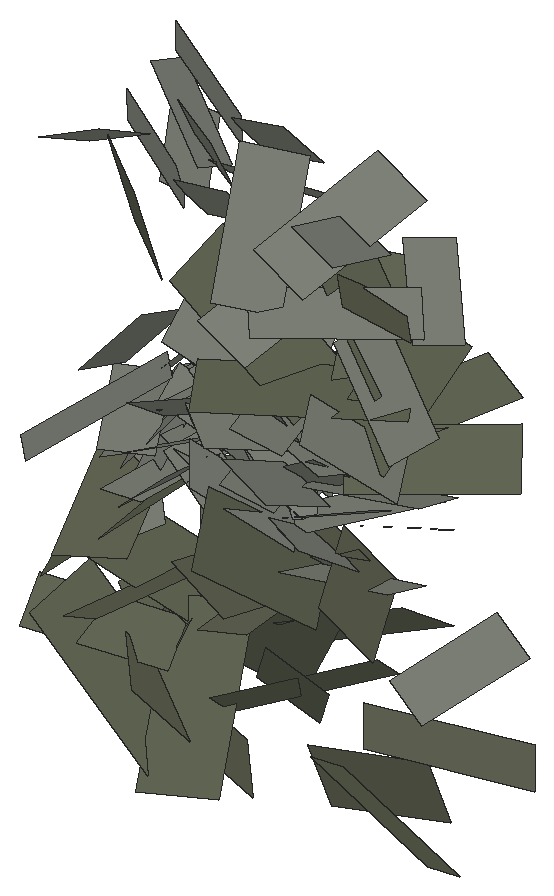
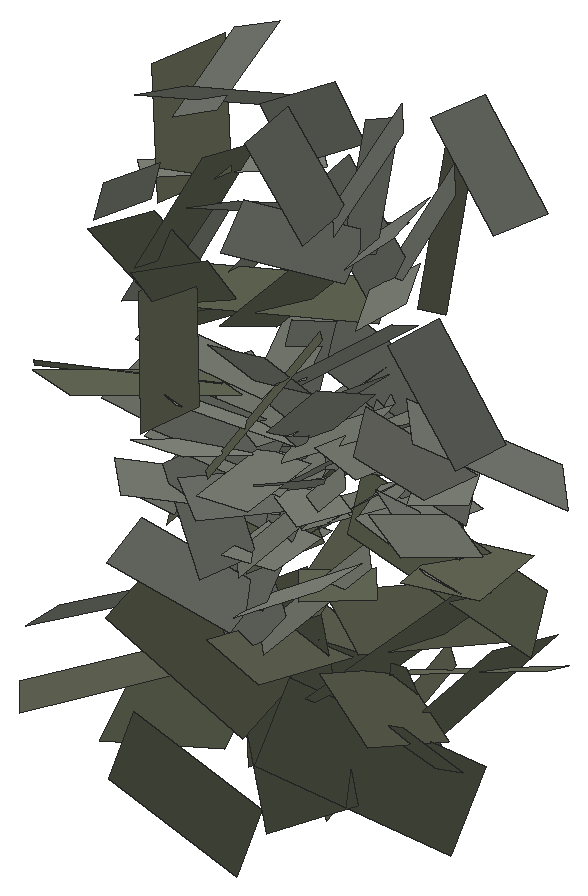
# SketchUp Ruby script. Lengths in inches.
U = 1.inch
M = Sketchup.active_model
def pt(a) = Geom::Point3d.new(a.map { |v| v * U })
def face(e, loops, mat)
  f = e.add_face(loops[0].map { |a| pt(a) })
  loops[1..].each { |l| e.add_face(l.map { |a| pt(a) }).erase! }
  f.material = f.back_material = mat if mat
  f
end
# faces: each face lists its corners as indices into pts; further lists are holes
def faces(e, pts, list, mat = nil) = list.each { |f| face(e, (f[0].is_a?(Array) ? f : [f]).map { |l| l.map { |i| pts[i] } }, mat) }
# xy, xz, yz: faces in a plane at the given z, y or x. An outline is a flat list of corners, or four numbers for a rectangle; further outlines are holes
def ring(l) = l.size == 4 ? [[l[0], l[1]], [l[2], l[1]], [l[2], l[3]], [l[0], l[3]]] : l.each_slice(2).to_a
def flat(e, list, mat, &to3) = list.each { |f| face(e, (f[0].is_a?(Array) ? f : [f]).map { |l| ring(l).map { |u, v| to3.(u, v) } }, mat) }
def xy(e, z, list, mat = nil) = flat(e, list, mat) { |x, y| [x, y, z] }
def xz(e, y, list, mat = nil) = flat(e, list, mat) { |x, z| [x, y, z] }
def yz(e, x, list, mat = nil) = flat(e, list, mat) { |y, z| [x, y, z] }
def lines(e, pts, list) = list.each { |a, b| e.add_line(pt(pts[a]), pt(pts[b])) }
# prism: a flat outline (further loops are holes) pulled along v
def prism(e, loops, v, mat = nil)
  f = face(e, loops, mat); d = Geom::Vector3d.new(v.map { |x| x * U })
  f.pushpull(f.normal.samedirection?(d) ? d.length : -d.length)
end
def box(e, o, s, mat = nil) = prism(e, [[o, [o[0] + s[0], o[1], o[2]], [o[0] + s[0], o[1] + s[1], o[2]], [o[0], o[1] + s[1], o[2]]]], [0, 0, s[2]], mat)
def at(x, y, z, deg = 0) = Geom::Transformation.translation(pt([x, y, z])) * Geom::Transformation.rotation(ORIGIN, Z_AXIS, deg.degrees)
def axes(o, x, y, z) = Geom::Transformation.new([*x, 0, *y, 0, *z, 0, *pt(o).to_a, 1])
def part(name) = M.definitions.add(name)
# library, detail: a bought-in or finely detailed component or shape, given as its bounding box
def library(name, o, s) = part(name).tap { |d| box(d.entities, o, s) }
def detail(e, o, s) = box(e.add_group.entities, o, s)
def put(e, d, t, mat = nil) = e.add_instance(d, t).tap { |i| i.material = mat if mat }
def group(e, t, mat = nil) = e.add_group.tap { |g| g.transformation = t; g.material = mat if mat }.entities
root = M.entities
M.materials.add("viburnumblaasdfas0df1w06d").color = [98, 102, 84]
M.materials.add("viburnumbladsadfasdfad0w122").color = [125, 129, 119]
c1 = part("Component\#315")
p = [[0.25,0,0],[2.05,0.01,0.35],[1.81,4.2,1.66],[0,4.19,1.3125]]
faces(c1.entities,p,[[0,1,2,3]],"viburnumbladsadfasdfad0w122")
c2 = part("viburnumblad2")
put(c2.entities,c1,axes([-19.23,-4.49,-32.18],[83.35428,0,0],[0,79.38502,0],[0,0,83.35428]))
c3 = part("Component\#314")
p = [[0.14,0,0],[2.58,0.05,0.25],[2.44,5.11,2.64],[0,5.05,2.39]]
faces(c3.entities,p,[[0,1,2,3]],"viburnumblaasdfas0df1w06d")
c4 = part("viburnumblad1\#2")
put(c4.entities,c3,axes([-37.25,6.23,19.31],[75.98784,0,0],[0,65.50676,0],[0,0,75.98784]))
put(root,c2,axes([1228.44,286.27,16.52],[0.01089,-0.00213,0.00325],[0.002,0.01232,0.0014],[-0.00372,-0.00076,0.01198]))
put(root,c2,axes([1227.97,286.51,28.15],[-0.00597,-0.01037,0.00113],[0.01154,-0.00613,0.0032],[-0.00222,0.00293,0.01099]))
put(root,c2,axes([1226.95,284.02,17.86],[0.01077,-0.01075,-0.00083],[0.01118,0.01095,0.00335],[-0.00168,-0.00283,0.01488]))
put(root,c2,axes([1230.21,287.73,26.82],[0.00649,0.00565,-0.00743],[-0.0085,0.00924,-0.00029],[0.00584,0.00584,0.00823]))
put(root,c4,axes([1229.8,282.66,14.06],[0.01294,0.00473,-0.00003],[-0.00539,0.01473,-0.00308],[-0.00088,0.0025,0.01352]))
put(root,c2,axes([1230.28,285.14,14.39],[0.0081,0.00545,0.00286],[-0.00642,0.00891,0.00123],[-0.00184,-0.00279,0.01054]))
put(root,c4,axes([1232.59,285.2,10],[-0.00341,0.01096,0.00392],[-0.01337,-0.00302,-0.00319],[-0.00164,-0.0045,0.01114]))
put(root,c2,axes([1230.37,283.98,18.52],[0.01038,0.0062,-0.0034],[-0.00717,0.01088,-0.00204],[0.00185,0.00346,0.01194]))
put(root,c2,axes([1231.46,287.4,26.4],[-0.00945,0.00892,-0.00145],[-0.0064,-0.00533,0.00736],[0.00487,0.007,0.00802]))
put(root,c2,axes([1231.55,287.99,27.68],[-0.00099,0.0108,-0.00603],[-0.01031,0.00186,0.00471],[0.00538,0.00602,0.00839]))
put(root,c2,axes([1228.79,287.2,19.83],[-0.00259,-0.01229,0.00001],[0.0107,-0.00225,0.00618],[-0.00604,0.00128,0.01094]))
put(root,c2,axes([1228.44,287.14,17.97],[0.0062,-0.01038,0.0034],[0.00931,0.00714,0.00482],[-0.00586,0.00014,0.01111]))
put(root,c4,axes([1232.05,286.2,7.57],[0.00865,0.00658,0.00734],[-0.00992,0.01145,0.00143],[-0.0049,-0.0056,0.0108]))
put(root,c4,axes([1227.57,284.9375,12.29],[0.0081,-0.01447,0.00211],[0.01627,0.00971,0.00411],[-0.00412,0.00005,0.0162]))
put(root,c2,axes([1229.75,285.68,15.67],[0.01032,-0.0026,0.00299],[0.00135,0.01024,0.00424],[-0.00373,-0.00356,0.00978]))
put(root,c4,axes([1230.71,285.7,8.77],[0.01224,-0.00166,0.00834],[0.00122,0.01717,0.00163],[-0.00844,-0.00056,0.01227]))
put(root,c4,axes([1230.86,286.15,23.78],[-0.01166,0.00571,0.00452],[-0.00151,-0.01177,0.01017],[0.0071,0.00732,0.00793]))
put(root,c4,axes([1233.14,284.03,6.07],[0.00022,0.01682,0.00237],[-0.01794,-0.00091,0.00812],[0.00704,-0.00224,0.0153]))
put(root,c4,axes([1228.48,287.45,6.375],[0.00095,-0.01143,0.01095],[0.01752,0.00456,0.00324],[-0.00472,0.01026,0.01113]))
put(root,c4,axes([1233.08,288.2,9.65],[-0.00358,0.0126,0.00711],[-0.01496,-0.00708,0.005],[0.00656,-0.00511,0.01237]))
put(root,c2,axes([1232.67,288.93,28.52],[-0.00905,0.00854,-0.00139],[-0.00711,-0.00593,0.00818],[0.00487,0.007,0.00802]))
put(root,c2,axes([1230.2,284.41,16.75],[0.01283,-0.0027,-0.00001],[0.00224,0.01066,-0.00301],[0.0007,0.00327,0.01211]))
put(root,c2,axes([1229.92,285.9375,17.31],[0.00604,-0.00926,0.00001],[0.00806,0.00526,0.00544],[-0.00456,-0.00296,0.00963]))
put(root,c4,axes([1229.6,283.08,11.54],[0.01155,-0.00606,0.00446],[0.00831,0.01316,-0.00362],[-0.00229,0.00493,0.01266]))
put(root,c2,axes([1230.25,285.44,19.69],[0.01229,-0.00259,-0.00001],[0.00249,0.01185,-0.00335],[0.0007,0.00327,0.01211]))
put(root,c2,axes([1232.37,288.87,26.84],[-0.01181,0.00128,0.00407],[0.00154,-0.01046,0.00743],[0.00382,0.0075,0.00815]))
put(root,c2,axes([1230.95,286.21,16.21],[-0.00178,-0.0105,-0.00298],[0.00981,-0.00286,0.00422],[-0.00478,-0.00196,0.00978]))
put(root,c2,axes([1230.54,285.33,17.9375],[0.007,-0.00987,0.00339],[0.00957,0.00618,-0.0018],[-0.00027,0.0039,0.01194]))
put(root,c2,axes([1234.54,289.21,14.47],[0.00007,0.01222,-0.00309],[-0.01226,0.00091,0.00331],[0.0034,0.00296,0.01177]))
put(root,c2,axes([1231.44,288.74,25.56],[-0.00734,-0.00647,0.00686],[0.01022,-0.00834,0.00267],[0.00284,0.00722,0.00872]))
put(root,c4,axes([1233.8,285.51,13.37],[0.00989,0.00806,-0.00127],[-0.00946,0.01134,-0.00169],[0.00005,0.00193,0.01267]))
put(root,c4,axes([1234.6,286.67,5.19],[-0.01033,0.0106,0.00208],[-0.0106,-0.01173,0.00714],[0.00578,0.00298,0.01347]))
put(root,c2,axes([1234.88,287.15,17.48],[-0.00324,0.01089,0.00211],[-0.01127,-0.00408,0.00376],[0.00428,-0.00101,0.01177]))
put(root,c2,axes([1235.0625,286.23,16.13],[-0.00179,0.01029,-0.00409],[-0.01223,-0.00094,0.00298],[0.00221,0.00457,0.01052]))
put(root,c2,axes([1235.05,287.08,18.96],[-0.00186,0.01072,-0.00426],[-0.01132,-0.00087,0.00276],[0.00221,0.00457,0.01052]))
put(root,c4,axes([1233.03,283.23,5.98],[0.01503,0.00487,0.00033],[-0.00521,0.01551,0.00826],[0.00191,-0.00687,0.0141]))
put(root,c2,axes([1234.36,286.95,19.07],[0.00616,0.01091,0.00086],[-0.01009,0.00525,0.00563],[0.00448,-0.00342,0.01123]))
put(root,c2,axes([1235.2,289.14,12.91],[-0.0083,0.00785,-0.00197],[-0.00857,-0.00783,0.00492],[0.002,0.00498,0.01141]))
put(root,c2,axes([1234.42,286.84,17.47],[0.00682,0.00858,-0.00405],[-0.00975,0.00742,-0.00069],[0.00196,0.0036,0.01094]))
put(root,c2,axes([1231.69,285.99,19.34],[-0.00239,-0.01136,0.0048],[0.01232,-0.002,0.0014],[-0.0005,0.00498,0.01153]))
put(root,c2,axes([1231.43,289.91,26.63],[0.00099,-0.0108,0.00603],[0.0122,-0.00051,-0.00294],[0.0025,0.00634,0.00938]))
put(root,c2,axes([1235.61,285.54,14.84],[-0.00037,0.01298,-0.00224],[-0.01317,0.00059,0.00559],[0.0056,0.0024,0.01296]))
put(root,c2,axes([1235.53,289.9,15.8125],[-0.00876,0.00902,-0.0009],[-0.00857,-0.00783,0.00492],[0.00296,0.00403,0.01157]))
put(root,c2,axes([1235.57,286.57,20.35],[-0.00304,0.01166,0.00355],[-0.01127,-0.00408,0.00376],[0.00464,-0.00228,0.01145]))
put(root,c2,axes([1232.8,290.25,27.68],[-0.00765,-0.00673,0.00714],[0.00947,-0.00772,0.00247],[0.00284,0.00722,0.00872]))
put(root,c4,axes([1232.87,290.7,6.53],[-0.01405,-0.00766,0.00571],[0.01107,-0.01374,0.00878],[0.00057,0.00947,0.0141]))
put(root,c2,axes([1235.74,286.91,17.37],[-0.00945,0.00658,-0.00199],[-0.00667,-0.00798,0.00533],[0.00164,0.00544,0.01021]))
put(root,c4,axes([1233.21,285.82,11.08],[0.01241,-0.00186,0.00262],[0.00291,0.01409,-0.00376],[-0.00201,0.00365,0.01212]))
put(root,c2,axes([1235.13,286.12,16.61],[0.00988,0.00976,-0.00351],[-0.00912,0.01058,0.00376],[0.00511,-0.00035,0.01338]))
put(root,c2,axes([1233.9375,287.17,15.875],[0.01201,0.00148,-0.00152],[-0.00157,0.01006,-0.00263],[0.00104,0.00309,0.01122]))
put(root,c2,axes([1234.02,288.09,18.62],[0.01151,0.00142,-0.00146],[-0.00175,0.01118,-0.00292],[0.00104,0.00309,0.01122]))
put(root,c4,axes([1234.72,288.91,12.13],[-0.01223,0.00026,0.00635],[-0.0009,-0.01592,-0.0011],[0.0063,-0.0012,0.0122]))
put(root,c2,axes([1236.49,285.88,18.14],[0.00021,0.01428,-0.00102],[-0.01317,0.00059,0.00559],[0.00561,0.00086,0.01315]))
put(root,c2,axes([1236.01,287.49,18.7],[-0.01046,0.00558,0.00416],[-0.00525,-0.01025,0.00054],[0.00396,-0.00141,0.01184]))
put(root,c4,axes([1236.1,290.48,18.02],[-0.00832,0.00937,0.00389],[-0.0091,-0.01059,0.00604],[0.00643,0.00098,0.01139]))
put(root,c2,axes([1234.4,287.5,20.88],[0.01175,0.00377,-0.00233],[-0.00262,0.01124,0.00497],[0.00358,-0.00416,0.0113]))
put(root,c2,axes([1235.79,290.36,13.95],[-0.01246,0.00054,0.00182],[0.00014,-0.01079,0.00417],[0.00189,0.00451,0.01162]))
put(root,c2,axes([1237.0625,286.04,16.01],[-0.00958,0.01044,0.00206],[-0.00856,-0.00879,0.00474],[0.00514,0.00211,0.0132]))
put(root,c4,axes([1237.41,285.89,20.64],[0.00084,0.01421,0.00442],[-0.01582,-0.0012,0.00687],[0.00595,-0.00438,0.01294]))
put(root,c2,axes([1235.65,288.26,17.42],[-0.01227,-0.00394,0.00243],[0.00307,-0.01072,-0.00188],[0.00284,-0.00132,0.01217]))
put(root,c2,axes([1236.1,288.01,18.5],[-0.01151,-0.00142,0.00146],[0.00195,-0.0101,0.00555],[0.00059,0.0057,0.01018]))
put(root,c2,axes([1234.1,288.08,16.97],[0.00945,-0.00658,0.00199],[0.00631,0.00831,-0.00248],[-0.00002,0.00335,0.01119]))
put(root,c2,axes([1234.2,288.5,19.48],[0.01046,-0.00558,-0.00416],[0.00651,0.0105,0.0023],[0.00246,-0.00407,0.01163]))
put(root,c2,axes([1235.36,290.42,12.46],[-0.00925,-0.00862,0.00362],[0.00803,-0.00772,0.00213],[0.00081,0.00412,0.01188]))
put(root,c4,axes([1235.23,288.83,7.27],[-0.01191,-0.00399,0.00577],[0.00688,-0.0137,0.00471],[0.00376,0.00597,0.01189]))
put(root,c4,axes([1236.82,287.36,12.36],[-0.00461,0.01011,0.01059],[-0.01024,-0.0125,0.00748],[0.01168,-0.00415,0.00905]))
put(root,c2,axes([1236.6,282.4,26.79],[0.00902,0.01086,-0.00673],[-0.00719,0.01113,0.00831],[0.01056,-0.0017,0.01141]))
put(root,c2,axes([1236.56,287.81,20.37],[-0.01175,-0.00377,0.00233],[0.00341,-0.01191,-0.00208],[0.00284,-0.00132,0.01217]))
put(root,c2,axes([1235.51,287.39,18.32],[0.01376,-0.00048,-0.00394],[0.00069,0.01429,0.00066],[0.00391,-0.00082,0.01375]))
put(root,c4,axes([1234.71,289.56,14.61],[-0.00859,-0.01039,0.00287],[0.01161,-0.0105,-0.00325],[0.004,0.00034,0.01318]))
put(root,c2,axes([1235.8125,291.41,15.39],[-0.00886,-0.00826,0.00347],[0.00892,-0.00858,0.00237],[0.00081,0.00412,0.01188]))
put(root,c2,axes([1234.38,289.1,17.92],[0.00292,-0.01119,-0.00341],[0.01302,0.00368,-0.00094],[0.00178,-0.0032,0.01202]))
put(root,c2,axes([1234.8,288.04,15.55],[0.00176,-0.01022,0.00282],[0.01152,0.00195,-0.00013],[-0.00039,0.00304,0.01127]))
put(root,c4,axes([1234.08,285.86,8.375],[0.00317,-0.01127,0.00742],[0.01555,0.00409,-0.00043],[-0.00159,0.00725,0.0117]))
put(root,c2,axes([1235.37,283.24,25.32],[0.01184,-0.00027,-0.00922],[0.00172,0.01671,0.00172],[0.00948,-0.00223,0.01224]))
put(root,c2,axes([1235.72,288.29,16.8],[-0.00682,-0.00858,0.00405],[0.00958,-0.00605,0.00332],[-0.00034,0.0052,0.01046]))
put(root,c2,axes([1234.68,291.35,13.89],[-0.00007,-0.01222,0.00309],[0.01323,-0.00017,-0.00035],[0.00036,0.00309,0.01221]))
put(root,c2,axes([1235.07,289.01,18.16],[0.00186,-0.01072,0.00426],[0.01152,0.00195,-0.00013],[-0.00059,0.00423,0.01088]))
put(root,c2,axes([1235.54,288.82,19.16],[-0.00616,-0.01091,-0.00086],[0.01132,-0.00616,-0.00282],[0.00193,-0.00206,0.01224]))
put(root,c4,axes([1234.46,290.12,9.36],[-0.00313,-0.01186,0.00638],[0.01559,-0.00367,0.00082],[0.00085,0.00636,0.01225]))
put(root,c2,axes([1237.92,286.87,17.65],[-0.01376,0.00048,0.00394],[0.00028,-0.01406,0.00269],[0.00396,0.00266,0.0135]))
put(root,c4,axes([1233.6,284.625,21.8],[0.00835,-0.01477,-0.00252],[0.01522,0.00998,-0.00805],[0.00724,0.00145,0.01548]))
put(root,c2,axes([1235.39,288.74,20.9],[0.00304,-0.01166,-0.00355],[0.01206,0.00341,-0.00087],[0.00178,-0.0032,0.01202]))
put(root,c2,axes([1235.43,287.92,16.41],[0.00958,-0.01044,-0.00206],[0.01029,0.0098,-0.00181],[0.00273,-0.00027,0.01406]))
put(root,c4,axes([1236.94,292.12,19.97],[-0.01002,-0.00367,0.00577],[0.0058,-0.01266,0.00203],[0.00466,0.00382,0.01053]))
put(root,c4,axes([1235.24,289.47,4.09],[-0.00376,-0.0039,0.01194],[0.01323,-0.00731,0.00178],[0.00528,0.01082,0.0052]))
put(root,c2,axes([1236.97,287.73,15.95],[-0.00988,-0.00976,0.00351],[0.01049,-0.01076,-0.00039],[0.00277,0.00219,0.01388]))
put(root,c2,axes([1235.64,287.86,14.51],[-0.0002,-0.01371,0.00098],[0.01527,-0.0004,-0.00242],[0.00226,0.00098,0.01411]))
put(root,c4,axes([1238.36,286.4375,21.39],[0.00971,0.0077,-0.00377],[-0.00736,0.01191,0.00523],[0.00557,-0.00177,0.01033]))
put(root,c2,axes([1237.53,283.51,28.62],[0.01234,-0.00028,-0.00961],[0.00159,0.01547,0.00159],[0.00948,-0.00223,0.01224]))
put(root,c2,axes([1236.94,288.38,17.84],[-0.00021,-0.01428,0.00102],[0.01414,-0.00037,-0.00224],[0.00226,0.00098,0.01411]))
put(root,c4,axes([1236.96,287.69,19.46],[0.01206,-0.00628,-0.00336],[0.00668,0.01448,-0.00311],[0.00388,0.00091,0.01211]))
put(root,c2,axes([1236.75,284.16,26.68],[0.00842,-0.01125,-0.00685],[0.01063,0.01127,-0.00543],[0.00843,-0.00165,0.01307]))
put(root,c4,axes([1240.42,286.2,22.41],[0.00107,0.01287,0.00071],[-0.01171,0.00034,0.00907],[0.0079,-0.00141,0.00892]))
put(root,c2,axes([1240.6,286.66,28.14],[-0.0126,0.00044,0.00361],[-0.00031,-0.0113,0.00032],[0.00347,0.00024,0.01207]))
put(root,c2,axes([1241.4,286.04,19.2],[-0.00545,0.00916,0.00529],[-0.00808,-0.00821,0.00589],[0.00818,-0.00089,0.00998]))
put(root,c4,axes([1238.97,288.31,14.45],[-0.00936,-0.00465,0.0096],[0.00338,-0.01554,-0.00424],[0.01026,-0.00044,0.00979]))
put(root,c4,axes([1237.26,287.47,6.97],[0.00066,-0.01186,0.00699],[0.01121,-0.00532,-0.01007],[0.0098,0.00532,0.0081]))
put(root,c4,axes([1238.84,285.4375,20.49],[0.01029,0.00428,-0.00658],[0.00078,0.01194,0.00879],[0.00737,-0.00649,0.00685]))
put(root,c2,axes([1241.5,285.48,20.85],[0.00288,0.01252,0.00147],[-0.00904,0.00098,0.00938],[0.00888,-0.00309,0.00888]))
put(root,c4,axes([1237.57,287.61,19.44],[0.00626,-0.00918,-0.00848],[0.01094,0.01129,-0.00412],[0.00772,-0.00395,0.00939]))
put(root,c2,axes([1241.47,286.83,24.9],[0.0051,0.01038,-0.00415],[-0.00729,0.00572,0.00502],[0.00694,0.00038,0.0084]))
put(root,c4,axes([1239.8125,287.61,25.15],[-0.01089,-0.0066,0.00527],[0.00777,-0.0139,-0.00135],[0.00514,0.00164,0.01268]))
put(root,c4,axes([1238.27,287.5625,9.32],[0.00753,-0.01126,-0.00255],[0.00884,0.00827,-0.01044],[0.00867,0.00351,0.01012]))
put(root,c2,axes([1240.53,287.01,11.74],[0.00716,-0.00025,-0.0097],[-0.0002,0.01356,-0.00049],[0.01011,0.00042,0.00745]))
